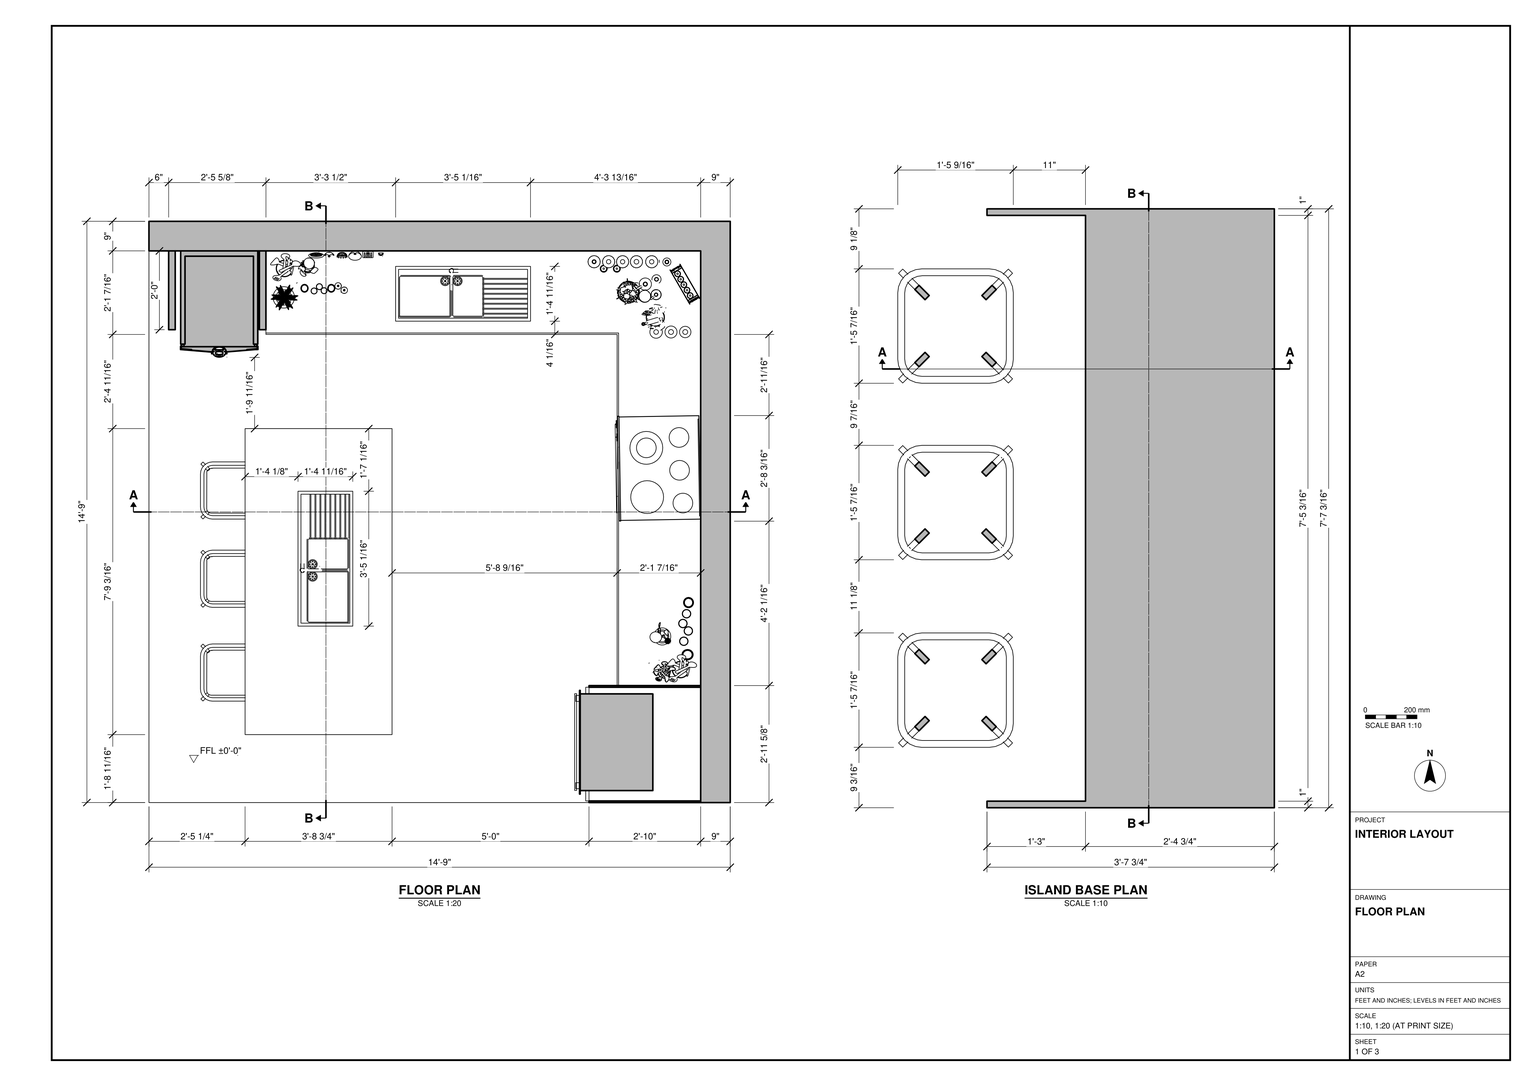
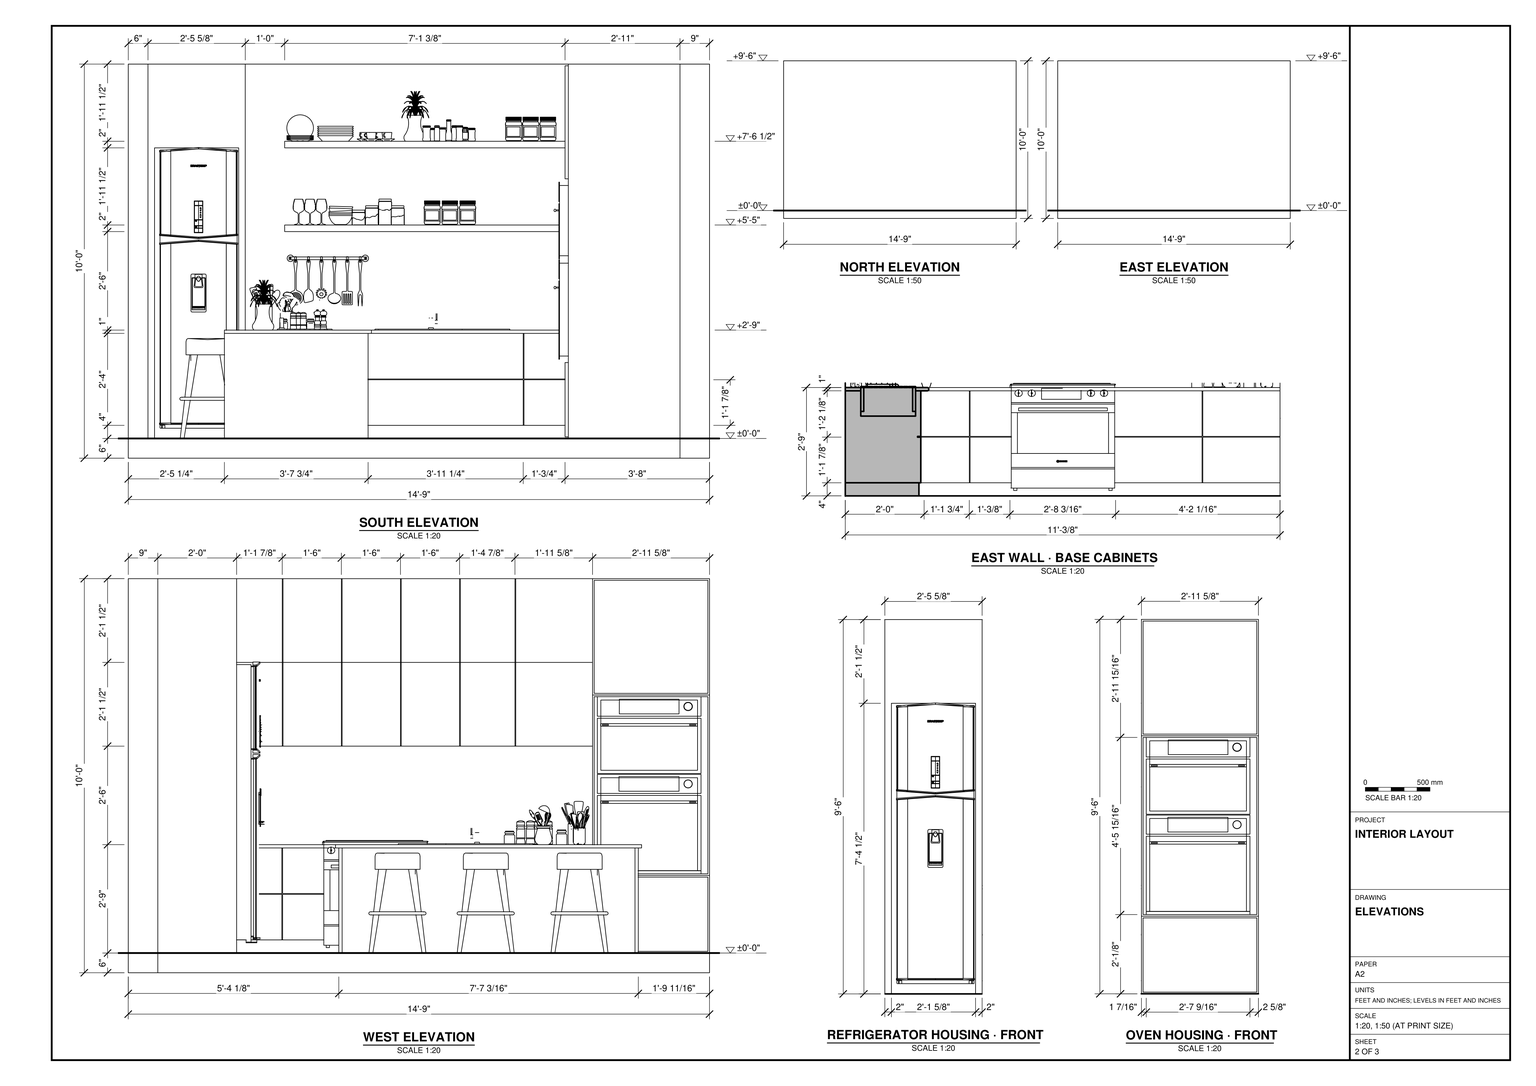
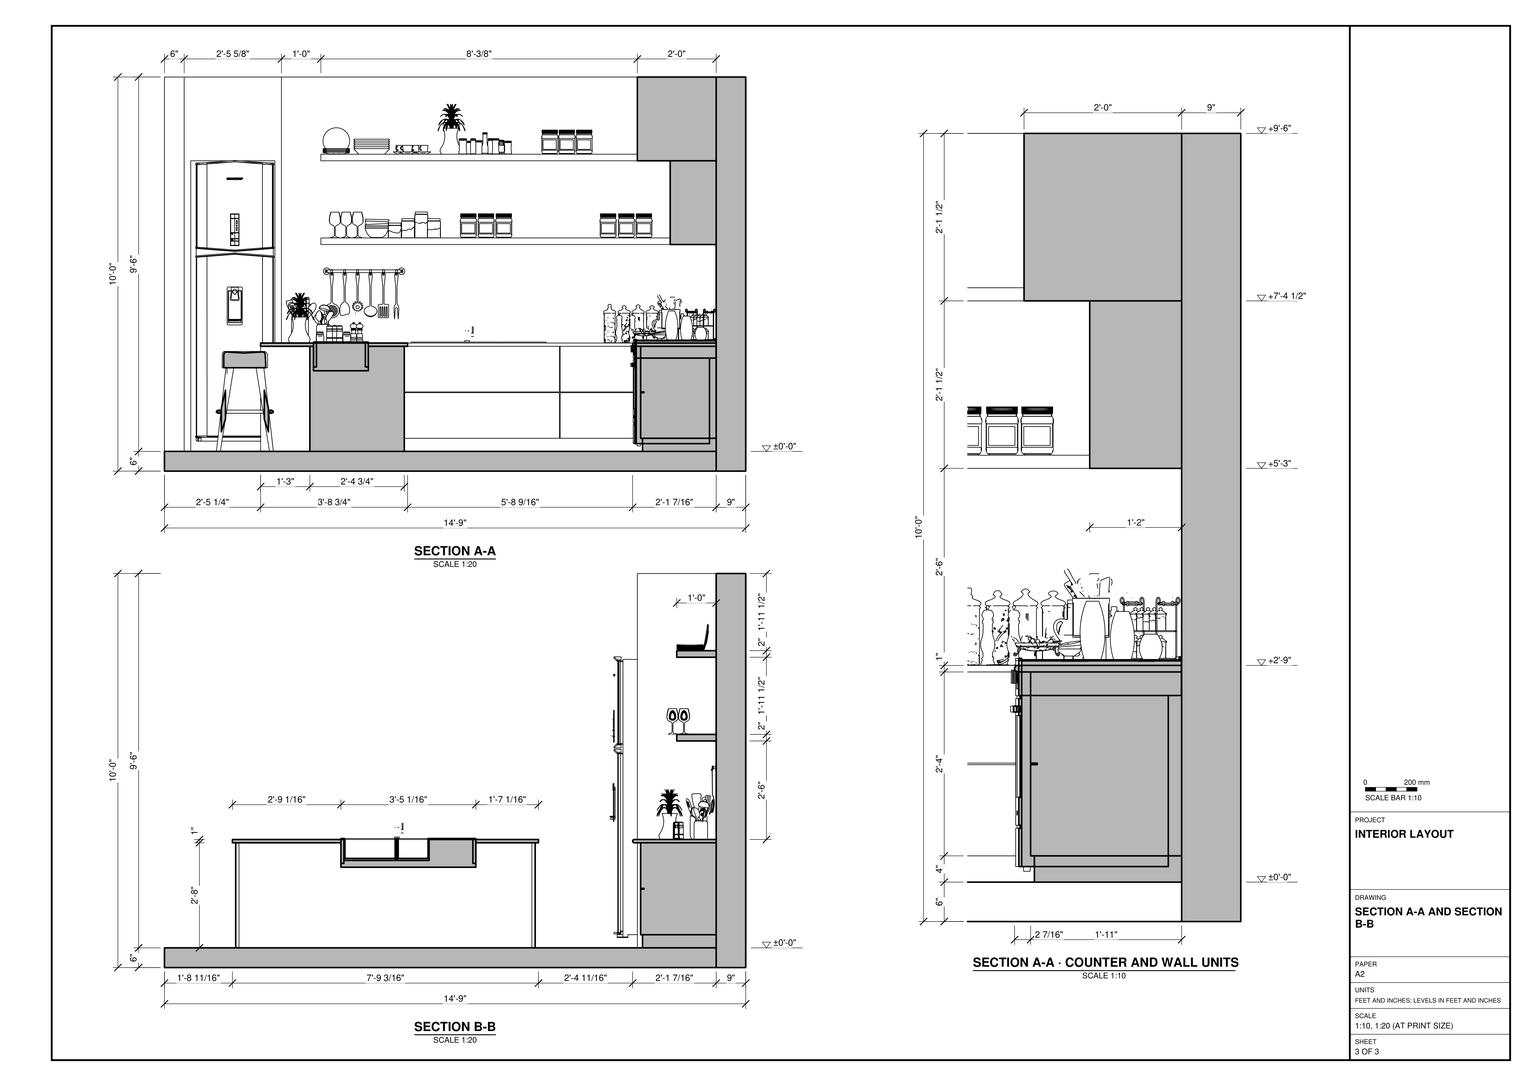
Build the kitchen in SketchUp from task_files/diagram_01.pdf. Work in feet and inches. The overall model is 14'-9" east to west, 14'-9" north to south and 10'-0" high. Set the finished floor at ±0'-0". Model the 6" floor slab and the 9" north and east walls, leaving the south and west sides open as drawn.

Fit the L-shaped cabinet run against the two walls. Use the elevations and sections to set the worktop height, recessed cabinet bases, front divisions and depths of the wall cabinets. Place the refrigerator housing at the west end of the north run and the stacked oven housing at the south end of the east run. Include the north counter sink and draining board, the open shelves and utensil rail above it, and the cooking unit in the east run.

Set out the island from the floor plan, using the separate base plan to distinguish its cabinet footprint from its worktop. Fit the second sink lengthwise in the island and leave knee space between the end panels for the three stools on the west side. Decor and loose items, including appliances, dishes, jars, plants and utensils, may be any suitable library components placed as shown.

Keep the slab, walls and individual joinery and furniture pieces in separate groups or components, and use components for repeated parts. Save one SketchUp model as output_files/l_shaped_kitchen_with_a_sink_island_and_seating.skp.

# SketchUp Ruby script. Lengths in inches.
U = 1.inch
M = Sketchup.active_model
def pt(a) = Geom::Point3d.new(a.map { |v| v * U })
def face(e, loops, mat)
  f = e.add_face(loops[0].map { |a| pt(a) })
  loops[1..].each { |l| e.add_face(l.map { |a| pt(a) }).erase! }
  f.material = f.back_material = mat if mat
  f
end
# faces: each face lists its corners as indices into pts; further lists are holes
def faces(e, pts, list, mat = nil) = list.each { |f| face(e, (f[0].is_a?(Array) ? f : [f]).map { |l| l.map { |i| pts[i] } }, mat) }
# xy, xz, yz: faces in a plane at the given z, y or x. An outline is a flat list of corners, or four numbers for a rectangle; further outlines are holes
def ring(l) = l.size == 4 ? [[l[0], l[1]], [l[2], l[1]], [l[2], l[3]], [l[0], l[3]]] : l.each_slice(2).to_a
def flat(e, list, mat, &to3) = list.each { |f| face(e, (f[0].is_a?(Array) ? f : [f]).map { |l| ring(l).map { |u, v| to3.(u, v) } }, mat) }
def xy(e, z, list, mat = nil) = flat(e, list, mat) { |x, y| [x, y, z] }
def xz(e, y, list, mat = nil) = flat(e, list, mat) { |x, z| [x, y, z] }
def yz(e, x, list, mat = nil) = flat(e, list, mat) { |y, z| [x, y, z] }
def lines(e, pts, list) = list.each { |a, b| e.add_line(pt(pts[a]), pt(pts[b])) }
# prism: a flat outline (further loops are holes) pulled along v
def prism(e, loops, v, mat = nil)
  f = face(e, loops, mat); d = Geom::Vector3d.new(v.map { |x| x * U })
  f.pushpull(f.normal.samedirection?(d) ? d.length : -d.length)
end
def box(e, o, s, mat = nil) = prism(e, [[o, [o[0] + s[0], o[1], o[2]], [o[0] + s[0], o[1] + s[1], o[2]], [o[0], o[1] + s[1], o[2]]]], [0, 0, s[2]], mat)
def at(x, y, z, deg = 0) = Geom::Transformation.translation(pt([x, y, z])) * Geom::Transformation.rotation(ORIGIN, Z_AXIS, deg.degrees)
def axes(o, x, y, z) = Geom::Transformation.new([*x, 0, *y, 0, *z, 0, *pt(o).to_a, 1])
def part(name) = M.definitions.add(name)
# library, detail: a bought-in or finely detailed component or shape, given as its bounding box
def library(name, o, s) = part(name).tap { |d| box(d.entities, o, s) }
def detail(e, o, s) = box(e.add_group.entities, o, s)
def put(e, d, t, mat = nil) = e.add_instance(d, t).tap { |i| i.material = mat if mat }
def group(e, t, mat = nil) = e.add_group.tap { |g| g.transformation = t; g.material = mat if mat }.entities
root = M.entities
M.materials.add("Material__5").color = [219, 188, 148]
M.materials.add("Material__8").color = [241, 238, 222]
M.materials.add("Material__9").color = [76, 62, 48]
M.materials.add("Paint-05").color = [0, 0, 0]
M.materials.add("Spice Bottle").color = [239, 229, 218]
M.materials.add("Wall").color = [252, 252, 252]
M.materials.add("[0011_Seashell]").color = [255, 245, 238]
M.materials.add("[0133_Gray]").color = [128, 128, 128]
M.materials.add("[Carrera Marble]").color = [207, 207, 207]
M.materials.add("[Field Rectangle Tile]").color = [196, 189, 179]
M.materials.add("[Granite Brown]").color = [126, 104, 91]
M.materials.add("[Tile Ceramic Multi]").color = [165, 115, 84]
M.materials.add("[Wood Floor Dark]").color = [153, 94, 42]
M.materials.add("[Wood Floor]").color = [155, 105, 61]
c1 = library("Untitled",[4.85,5.6,0],[28.36,32.44,74.22])
c2 = library("IKEA KULINARISK Ovens",[26.01,22.29,0],[23.39,23.8,41.3])
c3 = library("f0d72911-52da-47d9-be0f-e2779337d807",[0,0,0],[32.02,25.5625,36.34])
c4 = library("kitchen sink 48",[28.18,143.05,1.97],[53.35,21.66,22.86])
c5 = library("Group\#4",[-397.46,82.38,-0.11],[62.88,62.86,260])
c6 = library("Group\#5",[-282.65,82.375,-0.11],[62.85,62.875,260.02])
c7 = library("Group\#65",[222.96,189.98,-0.44],[259.48,39.25,337.49])
c8 = library("Group\#74",[41.52,-158.49,40.25],[95.93,90.14,172.87])
c9 = library("Group\#66",[-504.125,120.57,-0.1],[108.2,108.21,338.13])
c10 = library("Group\#67",[-376.9,120.94,-0.1],[107.79,107.8,326.37])
c11 = library("Group\#68",[-254.81,120.48,-0.6],[108.21,108.21,334.5])
c12 = library("Group\#69",[-133.01,121.19,-0.1],[106.95,106.95,324.89])
c13 = library("Group\#70",[0.46,121.12,-0.1],[106.94,106.94,338.14])
c14 = library("Group\#71",[151.35,137.54,-0.1],[70.51,70.14,256.45])
c15 = library("Group\#72",[-266.02,-201.27,40.23],[225.02,228.69,89.38])
c16 = library("Group\#73",[-78.56,-74.98,40.25],[131.28,107.59,245.3125])
c17 = library("Group\#75",[-60.55,-181.2,40.41],[105.85,106.35,65.49])
c18 = library("Group\#76",[253.59,42.68,151.97],[53.13,53.13,100.94])
c19 = library("Group\#77",[281.12,-5,151.97],[53.13,53.13,100.92])
c20 = library("Group\#78",[308.75,-52.85,151.97],[53.125,53.13,100.94])
c21 = library("Group\#79",[336.19,-100.38,151.98],[53.13,53.13,100.93])
c22 = library("Group\#80",[363.79,-148.1875,151.98],[53.13,53.13,100.93])
c23 = library("Group\#81",[253.59,42.68,30.7],[53.13,53.13,100.93])
c24 = library("Group\#82",[281.12,-5,30.7],[53.13,53.13,100.91])
c25 = library("Group\#83",[308.75,-52.85,30.7],[53.125,53.13,100.94])
c26 = library("Group\#84",[336.19,-100.38,30.7],[53.13,53.13,100.91])
c27 = library("Group\#85",[363.79,-148.1875,30.7],[53.13,53.13,100.93])
c28 = library("Group\#89",[212.54,-198.04,-0.24],[263.36,352.65,298.47])
c29 = library("Group\#90",[55.69,-19.19,40.37],[80.08,80.05,323.81])
c30 = part("SPICE")
p = [[1,1,0],[0,0,0],[1,0,0]]
lines(c30.entities,p,[[0,1],[1,2],[2,0]])
put(c30.entities,c5,at(0,0,0))
put(c30.entities,c6,at(0,0,0))
put(c30.entities,c7,at(0,0,0))
put(c30.entities,c8,at(0,0,0))
put(c30.entities,c9,at(0,0,0))
put(c30.entities,c10,at(0,0,0))
put(c30.entities,c11,at(0,0,0))
put(c30.entities,c12,at(0,0,0))
put(c30.entities,c13,at(0,0,0))
put(c30.entities,c14,at(0,0,0))
put(c30.entities,c15,at(0,0,0))
put(c30.entities,c16,at(0,0,0))
put(c30.entities,c17,at(0,0,0))
put(c30.entities,c18,at(0,0,0))
put(c30.entities,c19,at(0,0,0))
put(c30.entities,c20,at(0,0,0))
put(c30.entities,c21,at(0,0,0))
put(c30.entities,c22,at(0,0,0))
put(c30.entities,c23,at(0,0,0))
put(c30.entities,c24,at(0,0,0))
put(c30.entities,c25,at(0,0,0))
put(c30.entities,c26,at(0,0,0))
put(c30.entities,c27,at(0,0,0))
put(c30.entities,c28,at(0,0,0))
put(c30.entities,c29,at(0,0,0))
c31 = library("skpD5F4",[0,-2.85,-0.14],[24.79,2.85,15.53])
c32 = library("Wooden cutlery",[-2.99,-2.85,-0.03],[9.13,8.26,13.98])
c33 = library("0-25",[-52.18,-51.63,0],[103.29,103.26,236.65])
c34 = library("Encurtidos",[-8.17,-2.25,0],[16.27,5.07,6.57])
c35 = library("Decorative vase set",[0,0,0],[17.57,5.35,13.72])
c36 = library("Flacon épices",[-0.73,-0.83,0],[2.29,2.23,2.94])
c37 = library("~Epice",[-0.95,-0.95,0.13],[1.9,1.9,5.1])
c38 = library("~Tajine",[-0.52,-0.52,0],[2,2,6.24])
c39 = library("Utensils with color in holder",[0.34,2.72,-0.74],[8.53,8.52,13.22])
c40 = library("19 Kitchen",[-86.78,-82.07,0],[182.49,170.2,273.14])
c41 = library("barstool",[-0.12,-16.75,0],[17.59,17.42,30.4375])
c42 = part("Difference")
xy(c42.entities,0,[[[107.38,0,107.38,107.38,0,107.38,0,132.38,132.38,132.38,132.38,0],[39.49,110.97,80.57,127.66]]])
xy(c42.entities,0.01,[[107.31,0,107.31,107.31,107.34,107.34,107.34,0],[0,107.31,0,107.34,107.34,107.34,107.31,107.31]])
xy(c42.entities,0.99,[[107.31,0,107.34,0,107.34,107.34,107.31,107.31],[0,107.31,107.31,107.31,107.34,107.34,0,107.34]])
xy(c42.entities,1,[[[107.38,0,132.38,0,132.38,132.38,0,132.38,0,107.38,107.38,107.38],[39.49,110.97,80.57,127.66]]])
xz(c42.entities,0,[[107.38,0,132.38,0,132.38,1,107.38,1,107.34,0.99,107.31,0.99,107.27,0.97,107.24,0.96,107.21,0.94,107.18,0.93,107.15,0.91,107.12,0.88,107.09,0.86,107.07,0.83,107.04,0.8,107,0.74,106.99,0.71,106.97,0.68,106.96,0.64,106.95,0.61,106.95,0.57,106.94,0.54,106.94,0.46,106.95,0.43,106.95,0.39,106.96,0.36,106.97,0.32,106.99,0.29,107,0.26,107.04,0.2,107.07,0.17,107.09,0.14,107.12,0.12,107.15,0.09,107.18,0.07,107.21,0.06,107.24,0.04,107.27,0.03,107.31,0.01,107.34,0.01]])
xz(c42.entities,106.94,[[0,0.46,106.94,0.5],[0,0.5,106.94,0.54]])
xz(c42.entities,106.95,[[0,0.39,106.95,0.43],[0,0.57,106.95,0.61]])
xz(c42.entities,110.97,[[39.49,0,80.57,1]])
xz(c42.entities,127.66,[[39.49,0,80.57,1]])
xz(c42.entities,132.38,[[0,0,132.38,1]])
yz(c42.entities,0,[[107.38,0,107.34,0.01,107.31,0.01,107.27,0.03,107.24,0.04,107.21,0.06,107.18,0.07,107.15,0.09,107.12,0.12,107.09,0.14,107.07,0.17,107.04,0.2,107,0.26,106.99,0.29,106.97,0.32,106.96,0.36,106.95,0.39,106.95,0.43,106.94,0.46,106.94,0.54,106.95,0.57,106.95,0.61,106.96,0.64,106.97,0.68,106.99,0.71,107,0.74,107.04,0.8,107.07,0.83,107.09,0.86,107.12,0.88,107.15,0.91,107.18,0.93,107.21,0.94,107.24,0.96,107.27,0.97,107.31,0.99,107.34,0.99,107.38,1,132.38,1,132.38,0]])
yz(c42.entities,39.49,[[110.97,0,127.66,1]])
yz(c42.entities,80.57,[[110.97,0,127.66,1]])
yz(c42.entities,106.94,[[0,0.46,106.94,0.5],[0,0.5,106.94,0.54]])
yz(c42.entities,106.95,[[0,0.39,106.95,0.43],[0,0.57,106.95,0.61]])
yz(c42.entities,132.38,[[0,0,132.38,1]])
p = [[107.24,107.24,0.04],[107.27,107.27,0.03],[107.27,0,0.03],[107.24,0,0.04],[107.21,107.21,0.06],[107.21,0,0.06],
  [107.31,107.31,0.01],[107.31,0,0.01],[107.34,107.34,0.01],[107.38,107.38,0],[107.38,0,0],[107.34,0,0.01],
  [0,107.21,0.06],[0,107.24,0.04],[0,107.27,0.03],[0,107.31,0.01],[0,107.34,0.01],[0,107.38,0],
  [107.12,107.12,0.12],[107.15,107.15,0.09],[107.15,0,0.09],[107.12,0,0.12],[107.18,107.18,0.07],[107.18,0,0.07],
  [107.07,107.07,0.17],[107.09,107.09,0.14],[107.09,0,0.14],[107.07,0,0.17],[0,107.12,0.12],[0,107.15,0.09],
  [0,107.18,0.07],[0,107.07,0.17],[0,107.09,0.14],[107,107,0.26],[107.02,107.02,0.23],[107.02,0,0.23],
  [107,0,0.26],[107.04,107.04,0.2],[107.04,0,0.2],[0,107.02,0.23],[0,107.04,0.2],[0,107,0.26],
  [106.96,106.96,0.36],[106.97,106.97,0.32],[106.97,0,0.32],[106.96,0,0.36],[106.99,106.99,0.29],[106.99,0,0.29],
  [0,106.97,0.32],[0,106.99,0.29],[0,106.96,0.36],[106.94,106.94,0.46],[106.95,106.95,0.43],[106.95,0,0.43],
  [106.94,0,0.46],[106.95,106.95,0.39],[106.95,0,0.39],[0,106.94,0.46],[0,106.95,0.43],[0,106.95,0.39],
  [106.95,106.95,0.57],[106.94,106.94,0.54],[106.94,0,0.54],[106.95,0,0.57],[0,106.95,0.57],[0,106.94,0.54],
  [106.96,106.96,0.64],[106.95,106.95,0.61],[106.95,0,0.61],[106.96,0,0.64],[106.97,106.97,0.68],[106.97,0,0.68],
  [0,106.96,0.64],[0,106.95,0.61],[0,106.97,0.68],[107,107,0.74],[106.99,106.99,0.71],[106.99,0,0.71],
  [107,0,0.74],[107.02,107.02,0.77],[107.02,0,0.77],[0,107.02,0.77],[0,107,0.74],[0,106.99,0.71],
  [107.04,107.04,0.8],[107.04,0,0.8],[107.07,107.07,0.83],[107.07,0,0.83],[107.09,107.09,0.86],[107.09,0,0.86],
  [0,107.07,0.83],[0,107.04,0.8],[0,107.09,0.86],[107.18,107.18,0.93],[107.15,107.15,0.91],[107.15,0,0.91],
  [107.18,0,0.93],[107.12,107.12,0.88],[107.12,0,0.88],[107.21,107.21,0.94],[107.21,0,0.94],[107.24,107.24,0.96],
  [107.24,0,0.96],[0,107.12,0.88],[0,107.18,0.93],[0,107.15,0.91],[0,107.24,0.96],[0,107.21,0.94],
  [107.27,107.27,0.97],[107.27,0,0.97],[107.38,107.38,1],[107.34,107.34,0.99],[107.34,0,0.99],[107.38,0,1],
  [107.31,107.31,0.99],[107.31,0,0.99],[0,107.27,0.97],[0,107.31,0.99],[0,107.38,1],[0,107.34,0.99]]
faces(c42.entities,p,[[0,1,2,3],[4,0,3,5],[1,6,7,2],[8,9,10,11],[12,13,0,4],[13,14,1,0],[14,15,6,1],[16,17,9,8],
  [18,19,20,21],[19,22,23,20],[24,25,26,27],[25,18,21,26],[22,4,5,23],[28,29,19,18],[29,30,22,19],[31,32,25,24],
  [32,28,18,25],[30,12,4,22],[33,34,35,36],[34,37,38,35],[37,24,27,38],[39,40,37,34],[40,31,24,37],[41,39,34,33],
  [42,43,44,45],[43,46,47,44],[46,33,36,47],[48,49,46,43],[49,41,33,46],[50,48,43,42],[51,52,53,54],[55,42,45,56],
  [57,58,52,51],[59,50,42,55],[60,61,62,63],[64,65,61,60],[66,67,68,69],[70,66,69,71],[72,73,67,66],[74,72,66,70],
  [75,76,77,78],[76,70,71,77],[79,75,78,80],[81,82,75,79],[82,83,76,75],[83,74,70,76],[84,79,80,85],[86,84,85,87],
  [88,86,87,89],[90,91,84,86],[91,81,79,84],[92,90,86,88],[93,94,95,96],[94,97,98,95],[97,88,89,98],[99,93,96,100],
  [101,99,100,102],[103,92,88,97],[104,105,94,93],[105,103,97,94],[106,107,99,101],[107,104,93,99],[108,101,102,109],[110,111,112,113],
  [114,108,109,115],[116,106,101,108],[117,116,108,114],[118,119,111,110]])
c43 = part("Difference\#1")
xy(c43.entities,0,[[109.38,0,109.38,23.5,110.38,23.5,110.38,23.74,109.38,23.74,109.38,94.37,110.38,94.37,110.38,94.61,109.38,94.61,109.38,109.38,84.875,109.38,84.875,110.38,84.64,110.38,84.64,109.38,36.12,109.38,36.12,110.38,35.88,110.38,35.88,109.38,0,109.38,0,132.38,132.38,132.38,132.38,0]])
xy(c43.entities,13.88,[[109.38,0,110.38,23.5],[109.38,23.74,110.38,94.37],[109.38,94.61,110.38,94.61,110.38,110.38,84.875,110.38,84.875,109.38,109.38,109.38],[0,109.38,35.88,110.38],[36.12,109.38,84.64,110.38]])
xy(c43.entities,14.12,[[109.38,0,110.38,23.5],[109.38,23.74,110.38,94.37],[109.38,94.61,109.38,109.38,84.875,109.38,84.875,110.38,110.38,110.38,110.38,94.61],[0,109.38,35.88,110.38],[36.12,109.38,84.64,110.38]])
xy(c43.entities,20.3,[[39.49,110.97,80.57,127.66]])
xy(c43.entities,28,[[[109.38,0,132.38,0,132.38,132.38,0,132.38,0,109.38,35.88,109.38,35.88,110.38,36.12,110.38,36.12,109.38,84.64,109.38,84.64,110.38,84.875,110.38,84.875,109.38,109.38,109.38,109.38,94.61,110.38,94.61,110.38,94.37,109.38,94.37,109.38,23.74,110.38,23.74,110.38,23.5,109.38,23.5],[39.49,110.97,80.57,127.66]]])
xz(c43.entities,0,[[109.38,0,132.38,0,132.38,28,109.38,28,109.38,14.12,110.38,14.12,110.38,13.88,109.38,13.88]])
xz(c43.entities,23.5,[[109.38,0,110.38,13.88],[109.38,14.12,110.38,28]])
xz(c43.entities,23.74,[[109.38,0,110.38,13.88],[109.38,14.12,110.38,28]])
xz(c43.entities,94.37,[[109.38,0,110.38,13.88],[109.38,14.12,110.38,28]])
xz(c43.entities,94.61,[[109.38,0,110.38,13.88],[109.38,14.12,110.38,28]])
xz(c43.entities,109.38,[[0,0,35.88,13.88],[36.12,0,84.64,13.88],[84.875,0,109.38,13.88],[0,14.12,35.88,28],[36.12,14.12,84.64,28],
  [84.875,14.12,109.38,28]])
xz(c43.entities,110.38,[[35.88,0,36.12,0,36.12,13.88,84.64,13.88,84.64,0,84.875,0,84.875,13.88,110.38,13.88,110.38,14.12,84.875,14.12,84.875,28,84.64,28,84.64,14.12,36.12,14.12,36.12,28,35.88,28,35.88,14.12,0,14.12,0,13.88,35.88,13.88]])
xz(c43.entities,110.97,[[39.49,20.3,80.57,28]])
xz(c43.entities,127.66,[[39.49,20.3,80.57,28]])
xz(c43.entities,132.38,[[0,0,132.38,28]])
yz(c43.entities,0,[[109.38,0,109.38,13.88,110.38,13.88,110.38,14.12,109.38,14.12,109.38,28,132.38,28,132.38,0]])
yz(c43.entities,35.88,[[109.38,0,110.38,13.88],[109.38,14.12,110.38,28]])
yz(c43.entities,36.12,[[109.38,0,110.38,13.88],[109.38,14.12,110.38,28]])
yz(c43.entities,39.49,[[110.97,20.3,127.66,28]])
yz(c43.entities,80.57,[[110.97,20.3,127.66,28]])
yz(c43.entities,84.64,[[109.38,0,110.38,13.88],[109.38,14.12,110.38,28]])
yz(c43.entities,84.875,[[109.38,0,110.38,13.88],[109.38,14.12,110.38,28]])
yz(c43.entities,109.38,[[0,0,23.5,13.88],[23.74,0,94.37,13.88],[94.61,0,109.38,13.88],[0,14.12,23.5,28],[23.74,14.12,94.37,28],
  [94.61,14.12,109.38,28]])
yz(c43.entities,110.38,[[23.5,0,23.5,13.88,0,13.88,0,14.12,23.5,14.12,23.5,28,23.74,28,23.74,14.12,94.37,14.12,94.37,28,94.61,28,94.61,14.12,110.38,14.12,110.38,13.88,94.61,13.88,94.61,0,94.37,0,94.37,13.88,23.74,13.88,23.74,0]])
yz(c43.entities,132.38,[[0,0,132.38,28]])
c44 = library("Group",[-80,-80,0],[160,160,233.55])
c45 = library("Group1",[-80,-80,-284.86],[160,160,314.86])
c46 = library("Group4",[-80,-80,0],[160,160,233.55])
c47 = library("Group6",[-80,-80,-150.48],[160,160,180.48])
c48 = library("Group\#96",[-1.4,-1.39,0],[10.05,9.93,5.77])
c49 = library("Group\#97",[0,0,0],[10.9,5.85,4.58])
c50 = library("Group\#98",[0,0,-0.07],[8.11,9.93,8.07])
c51 = library("Group\#99",[-0.94,-0.94,0],[13.25,11.21,2.7])
c52 = library("Group\#260",[0,0,0],[5,5,7.36])
c53 = library("Group\#315",[0,0,0],[5,5,7.36])
c54 = library("Group\#317",[0,0,0],[5,5,7.36])
c55 = library("Group\#301",[0,0,0],[8.34,8.34,12.27])
c56 = library("Group\#299",[0,0,0],[8.34,8.34,12.27])
c57 = library("Group\#257",[0,0,0],[5,5,7.36])
c58 = library("Group\#125",[0,0,0],[8.34,8.34,12.27])
c59 = library("Group\#308",[0,0,0],[8.34,8.34,12.27])
c60 = library("Group\#267",[0,0,0],[8.34,8.34,12.27])
c61 = library("Group\#262",[0,-0.72,0],[10.99,11.66,20.3125])
c62 = library("Group\#94",[162.6875,-473.8,0.53],[157.34,166.37,329.78])
c63 = library("Group\#461",[71.89,225.55,9.24],[72.84,192.61,312.16])
c64 = library("Group\#463",[-34.9375,314.61,9],[141.36,134.24,278.875])
c65 = library("Group\#462",[-17.25,263.37,0.36],[173.25,173.26,183.12])
c66 = library("Group\#465",[1.63,276.74,6.1],[110.99,158.97,236.96])
c67 = library("Group\#466",[-20.56,278.78,6.51],[106.99,64.23,269.53])
c68 = library("Group\#467",[-51.36,334.47,6.18],[109.65,62.51,292.8])
c69 = library("Group\#468",[92.41,285.83,7.34],[85.49,97.03,269.76])
c70 = library("Group\#469",[4.4375,388.3,12.85],[187.55,49.52,268.59])
c71 = library("Group\#470",[8.86,224.99,5.92],[54.39,202.66,262.27])
c72 = part("Difference\#2")
prism(c72.entities,[[[44.75,93.1875,0],[44.75,0,0],[0,0,0],[0,93.1875,0]],[[16.11,33.04,0],[32.79,33.04,0],[32.79,74.12,0],[16.11,74.12,0]]],[0,0,1])
c73 = part("Difference\#3")
xy(c73.entities,0,[[0,0,0,1,15,1,15,90.1875,0,90.1875,0,91.1875,43.75,91.1875,43.75,0]])
xy(c73.entities,24.55,[[16.11,32.04,32.79,73.12]])
xy(c73.entities,32,[[[0,0,43.75,0,43.75,91.1875,0,91.1875,0,90.1875,15,90.1875,15,1,0,1],[16.11,32.04,32.79,73.12]]])
xz(c73.entities,0,[[0,0,43.75,32]])
xz(c73.entities,1,[[0,0,15,32]])
xz(c73.entities,32.04,[[16.11,24.55,32.79,32]])
xz(c73.entities,73.12,[[16.11,24.55,32.79,32]])
xz(c73.entities,90.1875,[[0,0,15,32]])
xz(c73.entities,91.1875,[[0,0,43.75,32]])
yz(c73.entities,0,[[0,0,1,32],[90.1875,0,91.1875,32]])
yz(c73.entities,15,[[1,0,90.1875,32]])
yz(c73.entities,16.11,[[32.04,24.55,73.12,32]])
yz(c73.entities,32.79,[[32.04,24.55,73.12,32]])
yz(c73.entities,43.75,[[0,0,91.1875,32]])
put(root,c1,axes([5.42,129.96,9.12],[0.84,0,0],[0,1,0],[0,0,1.152]))
put(root,c2,axes([107.34,69.28,30.12],[0,-1.35,0],[1,0,0],[0,0,1.3062]))
put(root,c3,axes([141.91,117.6875,7.65],[0.01655,-0.99986,0],[0.99986,0.01655,0],[0,0,0.89819]))
put(root,c4,axes([53.41,36.45,30.21],[0.77,0,0],[0,0.77,0],[0,0,0.77]))
put(root,c30,axes([151.21,158.62,39.02],[0.0348,0,0],[0,0.0348,0],[0,0,0.0348]))
put(root,c31,at(48.38,168,46.49))
put(root,c32,at(40.02,161.75,39))
put(root,c32,at(160.625,39.61,38.24))
put(root,c33,axes([58.79,154.7,71.05],[-0.03299,0,0],[0,0.03299,0],[0,0,0.03299]))
put(root,c33,axes([55.32,158.21,71.05],[-0.03299,0,0],[0,0.03299,0],[0,0,0.03299]))
put(root,c33,axes([55.32,154.7,71.05],[-0.03299,0,0],[0,0.03299,0],[0,0,0.03299]))
put(root,c33,axes([58.79,158.21,71.05],[-0.03299,0,0],[0,0.03299,0],[0,0,0.03299]))
put(root,c33,axes([51.86,158.21,71.05],[-0.03299,0,0],[0,0.03299,0],[0,0,0.03299]))
put(root,c33,axes([51.86,154.7,71.05],[-0.03299,0,0],[0,0.03299,0],[0,0,0.03299]))
put(root,c34,at(97.58,161.51,96.5))
put(root,c35,axes([165.04,145.21,39],[-0.71227,0,0],[0,-0.71227,0],[0,0,0.71227]),"Spice Bottle")
put(root,c36,axes([163.91,61.49,39],[0,-1.4,0],[1.4,0,0],[0,0,1.4]))
put(root,c37,axes([163.69,57.51,39],[1.33883,-0.40932,0],[0.40932,1.33883,0],[0,0,1.4]))
put(root,c37,axes([162.59,54.53,39],[1.05659,-0.91848,0],[0.91848,1.05659,0],[0,0,1.4]))
put(root,c37,axes([164.24,52.27,39],[0,-1.4,0],[1.4,0,0],[0,0,1.4]))
put(root,c37,axes([162.87,49.13,39],[1.36941,0.29108,0],[-0.29108,1.36941,0],[0,0,1.4]))
put(root,c37,at(50.28,155.8,39.15,-107))
put(root,c36,axes([46.95,156.3,39.15],[1.005,0,0],[0,1.11644,0],[0,0,1.095]))
put(root,c37,at(51.89,157.1,39.15,36))
put(root,c36,axes([55.1,156.3,39.15],[1.005,0,0],[0,1.11644,0],[0,0,1.095]))
put(root,c36,axes([163.56,45.63,39],[0,-1.407,0],[1.56301,0,0],[0,0,1.533]))
put(root,c37,at(53.32,155.88,39.15,136))
put(root,c38,at(57.125,156.85,39))
put(root,c38,at(58.98,155.55,39))
put(root,c39,axes([152.96,44.22,39.6875],[0.91501,0.16629,0],[-0.16629,0.91501,0],[0,0,0.93]),"Wall")
put(root,c40,axes([156.82,39.69,39],[0.03685,0,0],[0,0.03685,0],[0,0,0.03685]))
put(root,c41,at(15.81,103.08,6))
put(root,c41,at(15.81,76.2,6))
put(root,c41,at(15.81,47.64,6))
put(root,c4,axes([172.22,32.04,30.21],[0,0.77,0],[-0.77,0,0],[0,0,0.77]))
g1 = group(root,at(12,12,0))
xy(g1,0,[[-12,-12,156,156]])
xy(g1,6,[[-12,-12,156,156]],"[Tile Ceramic Multi]")
xz(g1,-12,[[-12,0,156,6]])
xz(g1,156,[[-12,0,156,6]])
yz(g1,-12,[[-12,0,156,6]])
yz(g1,156,[[-12,0,156,6]])
g2 = group(root,at(35.62,35.62,6),"Paint-05")
prism(g2,[[[109.95,109.95,0],[0,109.95,0],[0,132.38,0],[132.38,132.38,0],[132.38,0,0],[109.95,0,0]]],[0,0,4])
g3 = group(root,at(144,35.62,94.5),"[0011_Seashell]")
prism(g3,[[[24,132.38,0],[24,0,0],[0,0,0],[0,23.39,0],[1,23.39,0],[1,23.62,0],[0,23.62,0],[0,40.25,0],[1,40.25,0],[1,40.49,0],[0,40.49,0],[0,58.25,0],[1,58.25,0],[1,58.49,0],[0,58.49,0],[0,76.25,0],[1,76.25,0],[1,76.49,0],[0,76.49,0],[0,94.25,0],[1,94.25,0],[1,94.49,0],[0,94.49,0],[0,109.26,0],[1,109.26,0],[1,109.5,0],[11,109.5,0],[11,132.38,0]]],[0,0,25.5])
g4 = group(root,at(155,35.62,69),"[0011_Seashell]")
prism(g4,[[[13,132.38,0],[13,0,0],[-1,0,0],[-1,23.39,0],[0,23.39,0],[0,23.62,0],[-1,23.62,0],[-1,40.25,0],[0,40.25,0],[0,40.37,0],[0,40.49,0],[-1,40.49,0],[-1,58.25,0],[0,58.25,0],[0,58.37,0],[0,58.49,0],[-1,58.49,0],[-1,76.25,0],[0,76.25,0],[0,76.37,0],[0,76.49,0],[-1,76.49,0],[-1,94.25,0],[0,94.25,0],[0,94.37,0],[0,94.49,0],[-1,94.49,0],[-1,109.26,0],[0,109.26,0],[0,109.38,0],[0,109.5,0],[0,132.38,0]]],[0,0,25.5])
g5 = group(root,at(47.62,156,69),"[Wood Floor Dark]")
box(g5,[0,0,0],[107.38,12,2])
g6 = group(root,at(47.62,156,94.5),"[Wood Floor Dark]")
box(g6,[0,0,0],[107.38,12,2])
g7 = group(root,at(12,144,6),"[0011_Seashell]")
prism(g7,[[[-6,24,114],[23.62,24,114],[23.62,24,0],[21.62,24,0],[21.62,24,88.5],[-4,24,88.5],[-4,24,0],[-6,24,0]]],[0,-24,0])
g8 = group(root,at(132,0,6),"[0011_Seashell]")
xy(g8,0,[[2,0,36,35.62]])
xy(g8,0.5,[[1,0.5,2,35.12]])
xy(g8,23.12,[[1,0.5,2,35.12]])
xy(g8,24.12,[[2,0.5,36,35.12]])
xy(g8,78.07,[[2,0.5,36,35.12]])
xy(g8,79.07,[[1,0.5,2,35.12]])
xy(g8,113.5,[[1,0.5,2,35.12]])
xy(g8,114,[[2,0,36,35.62]])
xz(g8,0,[[2,0,36,114]])
xz(g8,0.5,[[1,0.5,2,23.12],[2,24.12,36,78.07],[1,79.07,2,113.5]])
xz(g8,35.12,[[1,0.5,2,23.12],[2,24.12,36,78.07],[1,79.07,2,113.5]])
xz(g8,35.62,[[2,0,36,114]])
yz(g8,1,[[0.5,0.5,35.12,23.12],[0.5,79.07,35.12,113.5]])
yz(g8,2,[[[0,0,35.62,23.62],[0.5,0.5,35.12,23.12]],[[0,23.62,35.62,78.57],[0.5,24.12,35.12,78.07]],[[0,78.57,35.62,114],[0.5,79.07,35.12,113.5]]])
yz(g8,36,[[[0,0,35.62,114],[0.5,24.12,35.12,78.07]]])
put(root,c42,at(35.62,35.62,38),"[Granite Brown]")
put(root,c43,at(35.62,35.62,10),"[0133_Gray]")
put(root,c44,axes([74.16,157.66,71],[-0.0144,0.02057,0],[0.02057,0.0144,0],[0,0,0.02511]))
put(root,c45,axes([78.21,158.56,78.15],[-0.00436,-0.02473,0],[-0.02473,0.00436,0],[0,0,0.02511]))
put(root,c46,axes([82.06,157.06,71],[-0.0144,0.02057,0],[0.02057,0.0144,0],[0,0,0.02511]))
put(root,c47,axes([70.14,158.13,74.78],[-0.01614,0.01924,0],[0.01924,0.01614,0],[0,0,0.02511]))
put(root,c48,at(61.07,152.58,71))
put(root,c49,at(57.64,156,96.5))
put(root,c50,at(48.28,156,96.57))
put(root,c51,at(69.71,156.94,96.5))
put(root,c52,at(114.83,156,96.5),"Spice Bottle")
put(root,c53,at(120.03,156,96.5),"Spice Bottle")
put(root,c54,at(125.3,156,96.5),"Spice Bottle")
put(root,c55,axes([138.14,156,71],[0.6,0,0],[0,0.6,0],[0,0,0.6]),"Spice Bottle")
put(root,c56,axes([132.59,156,71],[0.6,0,0],[0,0.6,0],[0,0,0.6]),"Spice Bottle")
put(root,c57,at(143.5,156,71),"Spice Bottle")
put(root,c58,axes([90.04,158.09,71],[0.6,0,0],[0,0.6,0],[0,0,0.6]),"Spice Bottle")
put(root,c59,axes([100.83,158.09,71],[0.6,0,0],[0,0.6,0],[0,0,0.6]),"Spice Bottle")
put(root,c60,axes([95.4375,158.09,71],[0.6,0,0],[0,0.6,0],[0,0,0.6]),"Spice Bottle")
put(root,c61,axes([37.15,149.97,39],[0.75,0,0],[0,0.75,0],[0,0,0.75]),"Spice Bottle")
put(root,c62,axes([62.5625,171.75,38.73],[0,-0.036,0],[0.036,0,0],[0,0,0.036]))
g9 = group(root,at(150.125,151.73,43.28))
put(g9,c63,axes([-7.3125,-1.67,-0.01],[0,-0.0325,0],[0.0325,0,0],[0,0,0.0325]),"Material__5")
put(g9,c64,axes([-7.3125,-1.67,-0.01],[0,-0.0325,0],[0.0325,0,0],[0,0,0.0325]),"Material__9")
put(g9,c65,axes([-7.3125,-1.67,-0.01],[0,-0.0325,0],[0.0325,0,0],[0,0,0.0325]),"Material__8")
put(g9,c66,axes([-7.3125,-1.67,-0.01],[0,-0.0325,0],[0.0325,0,0],[0,0,0.0325]),"Material__9")
put(g9,c67,axes([-7.3125,-1.67,-0.01],[0,-0.0325,0],[0.0325,0,0],[0,0,0.0325]),"Material__9")
put(g9,c68,axes([-7.3125,-1.67,-0.01],[0,-0.0325,0],[0.0325,0,0],[0,0,0.0325]),"Material__5")
put(g9,c69,axes([-7.3125,-1.67,-0.01],[0,-0.0325,0],[0.0325,0,0],[0,0,0.0325]),"Material__5")
put(g9,c70,axes([-7.3125,-1.67,-0.01],[0,-0.0325,0],[0.0325,0,0],[0,0,0.0325]),"Material__5")
put(g9,c71,axes([-7.3125,-1.67,-0.01],[0,-0.0325,0],[0.0325,0,0],[0,0,0.0325]),"Material__5")
put(root,c61,axes([83.29,159.96,96.5],[0.75,0,0],[0,0.75,0],[0,0,0.75]),"Spice Bottle")
put(root,c72,at(29.27,20.69,38),"[Carrera Marble]")
put(root,c73,at(29.27,21.69,6),"[Wood Floor]")
g10 = group(root,at(0,0,0))
xy(g10,0,[[168,0,168,168,0,168,0,177,177,177,177,0]])
xy(g10,120,[[168,0,177,0,177,177,0,177,0,168,168,168]])
xz(g10,0,[[168,0,177,120]])
xz(g10,168,[[0,0,168,120]],"[Field Rectangle Tile]")
xz(g10,177,[[0,0,177,120]])
yz(g10,0,[[168,0,177,120]])
yz(g10,168,[[0,0,168,120]],"[Field Rectangle Tile]")
yz(g10,177,[[0,0,177,120]])
p = [[35.62,168,120],[35.62,168,39]]
lines(g10,p,[[0,1]])
